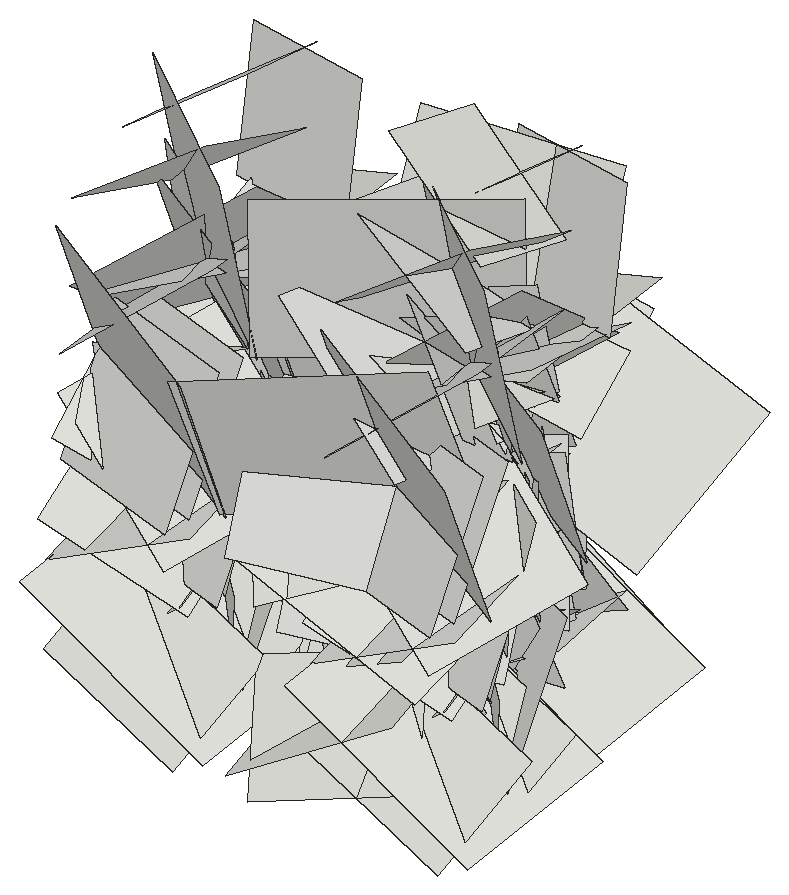
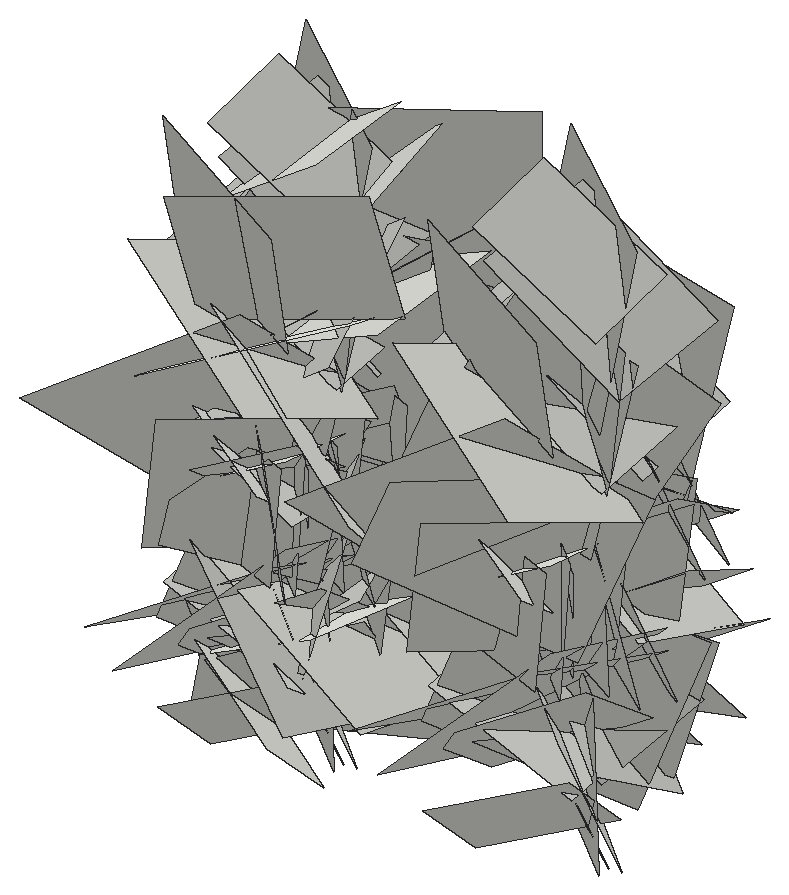
# SketchUp Ruby script. Lengths in inches.
U = 1.inch
M = Sketchup.active_model
def pt(a) = Geom::Point3d.new(a.map { |v| v * U })
def face(e, loops, mat)
  f = e.add_face(loops[0].map { |a| pt(a) })
  loops[1..].each { |l| e.add_face(l.map { |a| pt(a) }).erase! }
  f.material = f.back_material = mat if mat
  f
end
# faces: each face lists its corners as indices into pts; further lists are holes
def faces(e, pts, list, mat = nil) = list.each { |f| face(e, (f[0].is_a?(Array) ? f : [f]).map { |l| l.map { |i| pts[i] } }, mat) }
# xy, xz, yz: faces in a plane at the given z, y or x. An outline is a flat list of corners, or four numbers for a rectangle; further outlines are holes
def ring(l) = l.size == 4 ? [[l[0], l[1]], [l[2], l[1]], [l[2], l[3]], [l[0], l[3]]] : l.each_slice(2).to_a
def flat(e, list, mat, &to3) = list.each { |f| face(e, (f[0].is_a?(Array) ? f : [f]).map { |l| ring(l).map { |u, v| to3.(u, v) } }, mat) }
def xy(e, z, list, mat = nil) = flat(e, list, mat) { |x, y| [x, y, z] }
def xz(e, y, list, mat = nil) = flat(e, list, mat) { |x, z| [x, y, z] }
def yz(e, x, list, mat = nil) = flat(e, list, mat) { |y, z| [x, y, z] }
def lines(e, pts, list) = list.each { |a, b| e.add_line(pt(pts[a]), pt(pts[b])) }
# prism: a flat outline (further loops are holes) pulled along v
def prism(e, loops, v, mat = nil)
  f = face(e, loops, mat); d = Geom::Vector3d.new(v.map { |x| x * U })
  f.pushpull(f.normal.samedirection?(d) ? d.length : -d.length)
end
def box(e, o, s, mat = nil) = prism(e, [[o, [o[0] + s[0], o[1], o[2]], [o[0] + s[0], o[1] + s[1], o[2]], [o[0], o[1] + s[1], o[2]]]], [0, 0, s[2]], mat)
def at(x, y, z, deg = 0) = Geom::Transformation.translation(pt([x, y, z])) * Geom::Transformation.rotation(ORIGIN, Z_AXIS, deg.degrees)
def axes(o, x, y, z) = Geom::Transformation.new([*x, 0, *y, 0, *z, 0, *pt(o).to_a, 1])
def part(name) = M.definitions.add(name)
# library, detail: a bought-in or finely detailed component or shape, given as its bounding box
def library(name, o, s) = part(name).tap { |d| box(d.entities, o, s) }
def detail(e, o, s) = box(e.add_group.entities, o, s)
def put(e, d, t, mat = nil) = e.add_instance(d, t).tap { |i| i.material = mat if mat }
def group(e, t, mat = nil) = e.add_group.tap { |g| g.transformation = t; g.material = mat if mat }.entities
root = M.entities
c1 = part("Component\#6")
p = [[0.01,0,0],[0,3.24,4.54],[4.32,3.24,4.54],[4.33,0,0]]
faces(c1.entities,p,[[0,1,2,3]])
put(root,c1,axes([410.71,124,36.29],[-0.02149,0.52903,-1.24729],[0.2007,-1.23408,-0.5265],[1.42204,0.18216,0.05546]))
put(root,c1,axes([424.49,124,36.29],[0.02149,0.52903,-1.24729],[-0.2007,-1.23408,-0.5265],[-1.42204,0.18216,0.05546]))
put(root,c1,axes([420.52,124,36.29],[-0.02149,0.52903,-1.24729],[0.2007,-1.23408,-0.5265],[1.42204,0.18216,0.05546]))
put(root,c1,axes([410.66,123.49,22.43],[0.36857,0.54861,0.76203],[0.54406,0.56941,-0.64413],[0.83345,-0.61431,0.08349]))
put(root,c1,axes([424.54,123.49,22.43],[-0.36857,0.54861,0.76203],[-0.54406,0.56941,-0.64413],[-0.83345,-0.61431,0.08349]))
put(root,c1,axes([420.46,123.49,22.43],[0.36857,0.54861,0.76203],[0.54406,0.56941,-0.64413],[0.83345,-0.61431,0.08349]))
put(root,c1,axes([410.71,126.73,32.74],[-0.07983,-0.47542,-1.06148],[0.1788,-1.05692,0.46141],[1.21984,0.1238,-0.1371]))
put(root,c1,axes([424.49,126.73,32.74],[0.07983,-0.47542,-1.06148],[-0.1788,-1.05692,0.46141],[-1.21984,0.1238,-0.1371]))
put(root,c1,axes([420.52,126.73,32.74],[-0.07983,-0.47542,-1.06148],[0.1788,-1.05692,0.46141],[1.21984,0.1238,-0.1371]))
put(root,c1,axes([410.71,122.33,25.2],[0.14417,1.26196,0.33106],[0.05821,0.32703,-1.26913],[1.38172,-0.14545,0.01892]))
put(root,c1,axes([424.49,122.33,25.2],[-0.14417,1.26196,0.33106],[-0.05821,0.32703,-1.26913],[-1.38172,-0.14545,0.01892]))
put(root,c1,axes([420.52,122.33,25.2],[0.14417,1.26196,0.33106],[0.05821,0.32703,-1.26913],[1.38172,-0.14545,0.01892]))
put(root,c1,axes([410.71,127.85,32.74],[-0.07983,-0.47542,-1.06148],[0.1788,-1.05692,0.46141],[1.21984,0.1238,-0.1371]))
put(root,c1,axes([424.49,127.85,32.74],[0.07983,-0.47542,-1.06148],[-0.1788,-1.05692,0.46141],[-1.21984,0.1238,-0.1371]))
put(root,c1,axes([420.52,127.85,32.74],[-0.07983,-0.47542,-1.06148],[0.1788,-1.05692,0.46141],[1.21984,0.1238,-0.1371]))
put(root,c1,axes([410.71,128.39,27.01],[0.01413,-1.13969,-0.35832],[0.11214,-0.35581,1.13564],[1.2614,0.04439,-0.09695]))
put(root,c1,axes([420.52,128.39,27.01],[0.01413,-1.13969,-0.35832],[0.11214,-0.35581,1.13564],[1.2614,0.04439,-0.09695]))
put(root,c1,axes([424.49,128.39,27.01],[-0.01413,-1.13969,-0.35832],[-0.11214,-0.35581,1.13564],[-1.2614,0.04439,-0.09695]))
put(root,c1,axes([410,124.93,30.08],[0.69154,0.83647,0.57299],[0.50453,0.34895,-1.05134],[0.94895,-0.79509,0.14141]))
put(root,c1,axes([425.2,124.93,30.08],[-0.69154,0.83647,0.57299],[-0.50453,0.34895,-1.05134],[-0.94895,-0.79509,0.14141]))
put(root,c1,axes([419.81,124.93,30.08],[0.69154,0.83647,0.57299],[0.50453,0.34895,-1.05134],[0.94895,-0.79509,0.14141]))
put(root,c1,axes([420.52,128.06,26.23],[-0.10092,-0.80547,-0.37503],[-0.00485,-0.37672,0.81027],[0.94179,-0.08825,-0.03602]))
put(root,c1,axes([414.68,128.06,26.23],[0.10092,-0.80547,-0.37503],[0.00485,-0.37672,0.81027],[-0.94179,-0.08825,-0.03602]))
put(root,c1,axes([424.49,128.06,26.23],[0.10092,-0.80547,-0.37503],[0.00485,-0.37672,0.81027],[-0.94179,-0.08825,-0.03602]))
put(root,c1,axes([410.71,128.2,32.33],[0.15852,-1.12421,0.05612],[-0.12401,0.04078,1.12872],[1.18668,0.15444,0.11046]))
put(root,c1,axes([424.49,128.2,32.33],[-0.15852,-1.12421,0.05612],[0.12401,0.04078,1.12872],[-1.18668,0.15444,0.11046]))
put(root,c1,axes([420.52,128.2,32.33],[0.15852,-1.12421,0.05612],[-0.12401,0.04078,1.12872],[1.18668,0.15444,0.11046]))
put(root,c1,axes([410.66,125.55,22.43],[0.36857,0.54861,0.76203],[0.54406,0.56941,-0.64413],[0.83345,-0.61431,0.08349]))
put(root,c1,axes([424.54,125.55,22.43],[-0.36857,0.54861,0.76203],[-0.54406,0.56941,-0.64413],[-0.83345,-0.61431,0.08349]))
put(root,c1,axes([420.46,125.55,22.43],[0.36857,0.54861,0.76203],[0.54406,0.56941,-0.64413],[0.83345,-0.61431,0.08349]))
put(root,c1,axes([420.52,129.13,29.07],[-0.11411,-0.79222,-0.47459],[-0.01099,-0.47673,0.79815],[0.97884,-0.0977,-0.04636]))
put(root,c1,axes([414.68,129.13,29.07],[0.11411,-0.79222,-0.47459],[0.01099,-0.47673,0.79815],[-0.97884,-0.0977,-0.04636]))
put(root,c1,axes([424.49,129.13,29.07],[0.11411,-0.79222,-0.47459],[0.01099,-0.47673,0.79815],[-0.97884,-0.0977,-0.04636]))
put(root,c1,axes([410.71,128.47,40.0625],[0.15368,0.21217,-1.35934],[-0.08132,-1.3635,-0.221],[1.45608,-0.09854,0.13113]))
put(root,c1,axes([420.52,128.47,40.0625],[0.15368,0.21217,-1.35934],[-0.08132,-1.3635,-0.221],[1.45608,-0.09854,0.13113]))
put(root,c1,axes([424.49,128.47,40.0625],[-0.15368,0.21217,-1.35934],[0.08132,-1.3635,-0.221],[-1.45608,-0.09854,0.13113]))
put(root,c1,axes([410.71,129.14,29.25],[-0.07983,-0.47542,-1.06148],[0.1788,-1.05692,0.46141],[1.21984,0.1238,-0.1371]))
put(root,c1,axes([420.52,129.14,29.25],[-0.07983,-0.47542,-1.06148],[0.1788,-1.05692,0.46141],[1.21984,0.1238,-0.1371]))
put(root,c1,axes([424.49,129.14,29.25],[0.07983,-0.47542,-1.06148],[-0.1788,-1.05692,0.46141],[-1.21984,0.1238,-0.1371]))
put(root,c1,axes([410.71,126.77,21.87],[-0.10992,-0.34124,0.92241],[0.05569,0.92428,0.34784],[1.04103,-0.08548,0.07879]))
put(root,c1,axes([424.49,126.77,21.87],[0.10992,-0.34124,0.92241],[-0.05569,0.92428,0.34784],[-1.04103,-0.08548,0.07879]))
put(root,c1,axes([420.52,126.77,21.87],[-0.10992,-0.34124,0.92241],[0.05569,0.92428,0.34784],[1.04103,-0.08548,0.07879]))
put(root,c1,axes([410.71,129.34,35.47],[-0.09463,-0.94647,0.23979],[-0.00571,0.24126,0.95028],[1.03494,-0.08521,0.02717]))
put(root,c1,axes([420.52,129.34,35.47],[-0.09463,-0.94647,0.23979],[-0.00571,0.24126,0.95028],[1.03494,-0.08521,0.02717]))
put(root,c1,axes([424.49,129.34,35.47],[0.09463,-0.94647,0.23979],[0.00571,0.24126,0.95028],[-1.03494,-0.08521,0.02717]))
put(root,c1,axes([410.71,130.61,23.63],[-0.04049,-0.92661,-0.53015],[-0.18829,-0.51758,0.91743],[1.11583,-0.12096,0.13557]))
put(root,c1,axes([420.52,130.61,23.63],[-0.04049,-0.92661,-0.53015],[-0.18829,-0.51758,0.91743],[1.11583,-0.12096,0.13557]))
put(root,c1,axes([424.49,130.61,23.63],[0.04049,-0.92661,-0.53015],[0.18829,-0.51758,0.91743],[-1.11583,-0.12096,0.13557]))
put(root,c1,axes([410.71,126.5625,26.98],[-0.04661,-0.13743,1.04442],[0.16266,1.03335,0.14244],[1.10472,-0.15795,0.02309]))
put(root,c1,axes([424.49,126.5625,26.98],[0.04661,-0.13743,1.04442],[-0.16266,1.03335,0.14244],[-1.10472,-0.15795,0.02309]))
put(root,c1,axes([420.52,126.5625,26.98],[-0.04661,-0.13743,1.04442],[0.16266,1.03335,0.14244],[1.10472,-0.15795,0.02309]))
put(root,c1,axes([420.52,128.14,26.625],[-0.13018,-0.67547,0.62862],[-0.07474,0.63918,0.67304],[0.97523,-0.04118,0.13549]))
put(root,c1,axes([414.68,128.14,26.625],[0.13018,-0.67547,0.62862],[0.07474,0.63918,0.67304],[-0.97523,-0.04118,0.13549]))
put(root,c1,axes([424.49,128.14,26.625],[0.13018,-0.67547,0.62862],[0.07474,0.63918,0.67304],[-0.97523,-0.04118,0.13549]))
put(root,c1,axes([410.71,130.48,31.34],[-0.20009,-0.24055,-1.32848],[-0.01815,-1.34087,0.24522],[1.43098,-0.05064,-0.18264]))
put(root,c1,axes([420.52,130.48,31.34],[-0.20009,-0.24055,-1.32848],[-0.01815,-1.34087,0.24522],[1.43098,-0.05064,-0.18264]))
put(root,c1,axes([424.49,130.48,31.34],[0.20009,-0.24055,-1.32848],[0.01815,-1.34087,0.24522],[-1.43098,-0.05064,-0.18264]))
put(root,c1,axes([414.68,126.29,27.49],[0.18614,0.86586,-0.34095],[0.04817,-0.35453,-0.87695],[-0.98523,0.14625,-0.10729]))
put(root,c1,axes([420.52,126.29,27.49],[-0.18614,0.86586,-0.34095],[-0.04817,-0.35453,-0.87695],[0.98523,0.14625,-0.10729]))
put(root,c1,axes([424.49,126.29,27.49],[0.18614,0.86586,-0.34095],[0.04817,-0.35453,-0.87695],[-0.98523,0.14625,-0.10729]))
put(root,c1,axes([410.71,130.13,32.75],[0.05656,-1.14018,0.16245],[0.17438,0.16851,1.12862],[1.20828,0.02906,-0.17049]))
put(root,c1,axes([420.52,130.13,32.75],[0.05656,-1.14018,0.16245],[0.17438,0.16851,1.12862],[1.20828,0.02906,-0.17049]))
put(root,c1,axes([424.49,130.13,32.75],[-0.05656,-1.14018,0.16245],[-0.17438,0.16851,1.12862],[-1.20828,0.02906,-0.17049]))
put(root,c1,axes([410.71,128.45,36.29],[-0.02149,0.52903,-1.24729],[0.2007,-1.23408,-0.5265],[1.42204,0.18216,0.05546]))
put(root,c1,axes([424.49,128.45,36.29],[0.02149,0.52903,-1.24729],[-0.2007,-1.23408,-0.5265],[-1.42204,0.18216,0.05546]))
put(root,c1,axes([420.52,128.45,36.29],[-0.02149,0.52903,-1.24729],[0.2007,-1.23408,-0.5265],[1.42204,0.18216,0.05546]))
put(root,c1,axes([410.71,129.02,36.97],[-0.03047,0.19902,-0.90037],[0.05941,-0.89877,-0.20045],[0.97562,0.06094,-0.01591]))
put(root,c1,axes([420.52,129.02,36.97],[-0.03047,0.19902,-0.90037],[0.05941,-0.89877,-0.20045],[0.97562,0.06094,-0.01591]))
put(root,c1,axes([424.49,129.02,36.97],[0.03047,0.19902,-0.90037],[-0.05941,-0.89877,-0.20045],[-0.97562,0.06094,-0.01591]))
put(root,c1,axes([410.71,130.54,26.21],[-0.16316,0.13144,-1.2549],[-0.21583,-1.25022,-0.10597],[1.31994,-0.18819,-0.17245]))
put(root,c1,axes([424.49,130.54,26.21],[0.16316,0.13144,-1.2549],[0.21583,-1.25022,-0.10597],[-1.31994,-0.18819,-0.17245]))
put(root,c1,axes([420.52,130.54,26.21],[-0.16316,0.13144,-1.2549],[-0.21583,-1.25022,-0.10597],[1.31994,-0.18819,-0.17245]))
put(root,c1,axes([410.71,129.15,30.625],[-0.089,-0.93417,0.70597],[-0.20388,0.70917,0.91554],[1.22433,0.05019,0.20378]))
put(root,c1,axes([420.52,129.15,30.625],[-0.089,-0.93417,0.70597],[-0.20388,0.70917,0.91554],[1.22433,0.05019,0.20378]))
put(root,c1,axes([424.49,129.15,30.625],[0.089,-0.93417,0.70597],[0.20388,0.70917,0.91554],[-1.22433,0.05019,0.20378]))
put(root,c1,axes([410.71,132.16,25.41],[-0.07094,-0.60211,-1.2376],[-0.1162,-1.23279,0.6057],[1.45423,-0.12788,-0.01197]))
put(root,c1,axes([420.52,132.16,25.41],[-0.07094,-0.60211,-1.2376],[-0.1162,-1.23279,0.6057],[1.45423,-0.12788,-0.01197]))
put(root,c1,axes([424.49,132.16,25.41],[0.07094,-0.60211,-1.2376],[0.1162,-1.23279,0.6057],[-1.45423,-0.12788,-0.01197]))
put(root,c1,axes([410.71,130.09,30.86],[-0.13772,0.10296,-1.023],[-0.01142,-1.03121,-0.10242],[1.08979,0.0022,-0.13035]))
put(root,c1,axes([420.52,130.09,30.86],[-0.13772,0.10296,-1.023],[-0.01142,-1.03121,-0.10242],[1.08979,0.0022,-0.13035]))
put(root,c1,axes([424.49,130.09,30.86],[0.13772,0.10296,-1.023],[0.01142,-1.03121,-0.10242],[-1.08979,0.0022,-0.13035]))
put(root,c1,axes([410.71,130.39,37.85],[0.05885,-0.83818,0.13983],[-0.03078,0.13818,0.83979],[0.90022,0.05952,0.01957]))
put(root,c1,axes([420.52,130.39,37.85],[0.05885,-0.83818,0.13983],[-0.03078,0.13818,0.83979],[0.90022,0.05952,0.01957]))
put(root,c1,axes([424.49,130.39,37.85],[-0.05885,-0.83818,0.13983],[0.03078,0.13818,0.83979],[-0.90022,0.05952,0.01957]))
put(root,c1,axes([410.71,128.44,21.53],[-0.07533,-0.68545,1.00594],[-0.30491,0.98857,0.65329],[1.25377,0.19923,0.21932]))
put(root,c1,axes([420.52,128.44,21.53],[-0.07533,-0.68545,1.00594],[-0.30491,0.98857,0.65329],[1.25377,0.19923,0.21932]))
put(root,c1,axes([424.49,128.44,21.53],[0.07533,-0.68545,1.00594],[0.30491,0.98857,0.65329],[-1.25377,0.19923,0.21932]))
put(root,c1,axes([410.71,131.26,22.93],[0.10206,-0.4663,-0.72841],[0.02316,-0.73136,0.47108],[0.91647,0.07041,0.06921]))
put(root,c1,axes([420.52,131.26,22.93],[0.10206,-0.4663,-0.72841],[0.02316,-0.73136,0.47108],[0.91647,0.07041,0.06921]))
put(root,c1,axes([424.49,131.26,22.93],[-0.10206,-0.4663,-0.72841],[-0.02316,-0.73136,0.47108],[-0.91647,0.07041,0.06921]))
put(root,c1,axes([410.71,131.47,30.67],[0.19347,-0.24403,-0.96391],[-0.05093,-0.98104,0.23927],[1.05275,-0.00261,0.18872]))
put(root,c1,axes([420.52,131.47,30.67],[0.19347,-0.24403,-0.96391],[-0.05093,-0.98104,0.23927],[1.05275,-0.00261,0.18872]))
put(root,c1,axes([424.49,131.47,30.67],[-0.19347,-0.24403,-0.96391],[0.05093,-0.98104,0.23927],[-1.05275,-0.00261,0.18872]))
put(root,c1,axes([410.71,131.58,31.0625],[0.07279,0.01987,-1.05868],[-0.10279,-1.05633,-0.02611],[1.11768,-0.09844,0.06655]))
put(root,c1,axes([420.52,131.58,31.0625],[0.07279,0.01987,-1.05868],[-0.10279,-1.05633,-0.02611],[1.11768,-0.09844,0.06655]))
put(root,c1,axes([424.49,131.58,31.0625],[-0.07279,0.01987,-1.05868],[0.10279,-1.05633,-0.02611],[-1.11768,-0.09844,0.06655]))
put(root,c1,axes([410.71,131.52,23.18],[0.15485,-0.9106,-0.00305],[0.11373,0.01414,0.91588],[0.95852,0.14543,-0.10818]))
put(root,c1,axes([420.52,131.52,23.18],[0.15485,-0.9106,-0.00305],[0.11373,0.01414,0.91588],[0.95852,0.14543,-0.10818]))
put(root,c1,axes([424.49,131.52,23.18],[-0.15485,-0.9106,-0.00305],[-0.11373,0.01414,0.91588],[-0.95852,0.14543,-0.10818]))
put(root,c1,axes([410.71,127.05,26.22],[0.14417,1.26196,0.33106],[0.05821,0.32703,-1.26913],[1.38172,-0.14545,0.01892]))
put(root,c1,axes([424.49,127.05,26.22],[-0.14417,1.26196,0.33106],[-0.05821,0.32703,-1.26913],[-1.38172,-0.14545,0.01892]))
put(root,c1,axes([420.52,127.05,26.22],[0.14417,1.26196,0.33106],[0.05821,0.32703,-1.26913],[1.38172,-0.14545,0.01892]))
put(root,c1,axes([410.71,127.73,24.28],[-0.02979,0.75993,0.53946],[-0.00151,0.53967,-0.7603],[0.98786,0.02374,0.0151]))
put(root,c1,axes([424.49,127.73,24.28],[0.02979,0.75993,0.53946],[0.00151,0.53967,-0.7603],[-0.98786,0.02374,0.0151]))
put(root,c1,axes([420.52,127.73,24.28],[-0.02979,0.75993,0.53946],[-0.00151,0.53967,-0.7603],[0.98786,0.02374,0.0151]))
put(root,c1,axes([410.71,127.1,26.99],[-0.01407,1.25738,0.35681],[-0.29384,0.346,-1.2296],[1.35392,0.08816,-0.26315]))
put(root,c1,axes([424.49,127.1,26.99],[0.01407,1.25738,0.35681],[0.29384,0.346,-1.2296],[-1.35392,0.08816,-0.26315]))
put(root,c1,axes([420.52,127.1,26.99],[-0.01407,1.25738,0.35681],[-0.29384,0.346,-1.2296],[1.35392,0.08816,-0.26315]))
put(root,c1,axes([410.71,129.03,31.05],[0.04043,0.74356,0.04678],[0.07255,0.04314,-0.74161],[0.78639,-0.04221,0.06601]))
put(root,c1,axes([420.52,129.03,31.05],[0.04043,0.74356,0.04678],[0.07255,0.04314,-0.74161],[0.78639,-0.04221,0.06601]))
put(root,c1,axes([424.49,129.03,31.05],[-0.04043,0.74356,0.04678],[-0.07255,0.04314,-0.74161],[-0.78639,-0.04221,0.06601]))
put(root,c1,axes([410.71,134.48,33.76],[-0.26334,-1.11466,-0.41014],[0.1173,-0.43892,1.12584],[1.25351,-0.19309,-0.19152]))
put(root,c1,axes([424.49,134.48,33.76],[0.26334,-1.11466,-0.41014],[-0.1173,-0.43892,1.12584],[-1.25351,-0.19309,-0.19152]))
put(root,c1,axes([420.52,134.48,33.76],[-0.26334,-1.11466,-0.41014],[0.1173,-0.43892,1.12584],[1.25351,-0.19309,-0.19152]))
put(root,c1,axes([414.68,133.52,31.89],[0.15087,-0.04242,-1.05475],[0.23169,-1.04005,0.07132],[-1.09469,-0.22597,-0.13027]))
put(root,c1,axes([420.52,133.52,31.89],[-0.15087,-0.04242,-1.05475],[-0.23169,-1.04005,0.07132],[1.09469,-0.22597,-0.13027]))
put(root,c1,axes([424.49,133.52,31.89],[0.15087,-0.04242,-1.05475],[0.23169,-1.04005,0.07132],[-1.09469,-0.22597,-0.13027]))
put(root,c1,axes([410.71,129.22,21.54],[-0.01805,0.58513,0.55019],[0.06792,0.54955,-0.58247],[0.84865,-0.03153,0.05832]))
put(root,c1,axes([420.52,129.22,21.54],[-0.01805,0.58513,0.55019],[0.06792,0.54955,-0.58247],[0.84865,-0.03153,0.05832]))
put(root,c1,axes([424.49,129.22,21.54],[0.01805,0.58513,0.55019],[-0.06792,0.54955,-0.58247],[-0.84865,-0.03153,0.05832]))
put(root,c1,axes([420.52,129.75,30.06],[0.01937,0.49926,0.36665],[0.0577,0.36409,-0.4985],[0.65405,-0.04691,0.03312]))
put(root,c1,axes([414.68,129.75,30.06],[-0.01937,0.49926,0.36665],[-0.0577,0.36409,-0.4985],[-0.65405,-0.04691,0.03312]))
put(root,c1,axes([424.49,129.75,30.06],[-0.01937,0.49926,0.36665],[-0.0577,0.36409,-0.4985],[-0.65405,-0.04691,0.03312]))
put(root,c1,axes([410.71,133.17,39.1],[0.0845,-0.28698,-1.03421],[0.22383,-1.0126,0.29726],[1.11545,0.22493,0.0187]))
put(root,c1,axes([424.49,133.17,39.1],[-0.0845,-0.28698,-1.03421],[-0.22383,-1.0126,0.29726],[-1.11545,0.22493,0.0187]))
put(root,c1,axes([420.52,133.17,39.1],[0.0845,-0.28698,-1.03421],[0.22383,-1.0126,0.29726],[1.11545,0.22493,0.0187]))
put(root,c1,axes([410.71,128.43,31.91],[0.33386,1.00192,0.91989],[0.02581,0.93993,-1.03208],[1.44154,-0.24887,-0.19457]))
put(root,c1,axes([420.52,128.43,31.91],[0.33386,1.00192,0.91989],[0.02581,0.93993,-1.03208],[1.44154,-0.24887,-0.19457]))
put(root,c1,axes([424.49,128.43,31.91],[-0.33386,1.00192,0.91989],[-0.02581,0.93993,-1.03208],[-1.44154,-0.24887,-0.19457]))
put(root,c1,axes([420.52,130.92,26.67],[-0.06799,-0.20959,0.7931],[0.02884,0.79454,0.21217],[0.86907,-0.04277,0.05501]))
put(root,c1,axes([414.68,130.92,26.67],[0.06799,-0.20959,0.7931],[-0.02884,0.79454,0.21217],[-0.86907,-0.04277,0.05501]))
put(root,c1,axes([424.49,130.92,26.67],[0.06799,-0.20959,0.7931],[-0.02884,0.79454,0.21217],[-0.86907,-0.04277,0.05501]))
put(root,c1,axes([410.71,131.21,27.63],[-0.2234,-0.54463,1.08834],[-0.02633,1.10624,0.54877],[1.28976,-0.07175,0.19972]))
